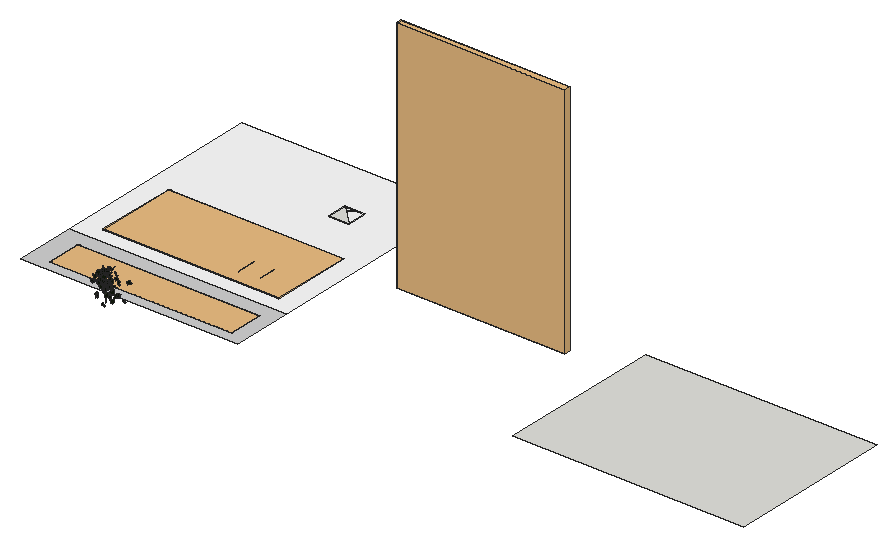
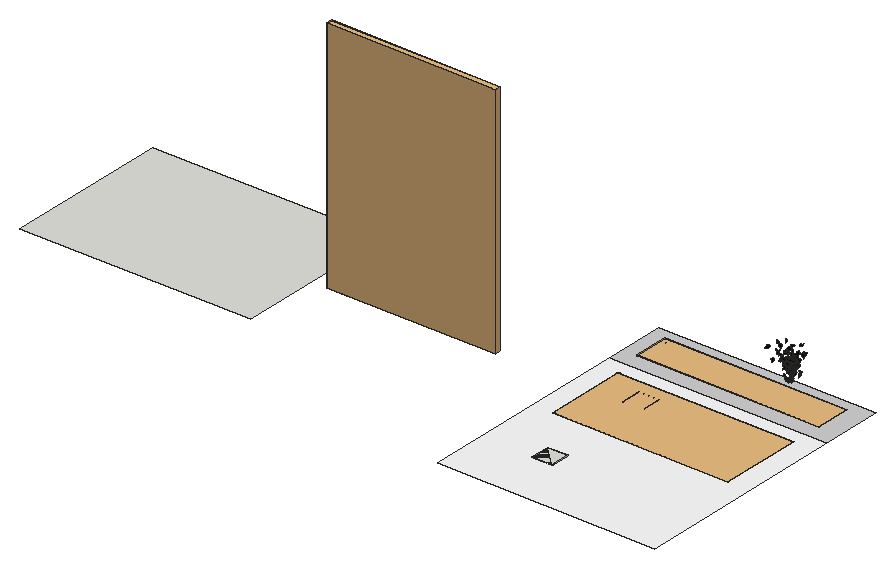
# SketchUp Ruby script. Lengths in inches.
U = 1.inch
M = Sketchup.active_model
def pt(a) = Geom::Point3d.new(a.map { |v| v * U })
def face(e, loops, mat)
  f = e.add_face(loops[0].map { |a| pt(a) })
  loops[1..].each { |l| e.add_face(l.map { |a| pt(a) }).erase! }
  f.material = f.back_material = mat if mat
  f
end
# faces: each face lists its corners as indices into pts; further lists are holes
def faces(e, pts, list, mat = nil) = list.each { |f| face(e, (f[0].is_a?(Array) ? f : [f]).map { |l| l.map { |i| pts[i] } }, mat) }
# xy, xz, yz: faces in a plane at the given z, y or x. An outline is a flat list of corners, or four numbers for a rectangle; further outlines are holes
def ring(l) = l.size == 4 ? [[l[0], l[1]], [l[2], l[1]], [l[2], l[3]], [l[0], l[3]]] : l.each_slice(2).to_a
def flat(e, list, mat, &to3) = list.each { |f| face(e, (f[0].is_a?(Array) ? f : [f]).map { |l| ring(l).map { |u, v| to3.(u, v) } }, mat) }
def xy(e, z, list, mat = nil) = flat(e, list, mat) { |x, y| [x, y, z] }
def xz(e, y, list, mat = nil) = flat(e, list, mat) { |x, z| [x, y, z] }
def yz(e, x, list, mat = nil) = flat(e, list, mat) { |y, z| [x, y, z] }
def lines(e, pts, list) = list.each { |a, b| e.add_line(pt(pts[a]), pt(pts[b])) }
# prism: a flat outline (further loops are holes) pulled along v
def prism(e, loops, v, mat = nil)
  f = face(e, loops, mat); d = Geom::Vector3d.new(v.map { |x| x * U })
  f.pushpull(f.normal.samedirection?(d) ? d.length : -d.length)
end
def box(e, o, s, mat = nil) = prism(e, [[o, [o[0] + s[0], o[1], o[2]], [o[0] + s[0], o[1] + s[1], o[2]], [o[0], o[1] + s[1], o[2]]]], [0, 0, s[2]], mat)
def at(x, y, z, deg = 0) = Geom::Transformation.translation(pt([x, y, z])) * Geom::Transformation.rotation(ORIGIN, Z_AXIS, deg.degrees)
def axes(o, x, y, z) = Geom::Transformation.new([*x, 0, *y, 0, *z, 0, *pt(o).to_a, 1])
def part(name) = M.definitions.add(name)
# library, detail: a bought-in or finely detailed component or shape, given as its bounding box
def library(name, o, s) = part(name).tap { |d| box(d.entities, o, s) }
def detail(e, o, s) = box(e.add_group.entities, o, s)
def put(e, d, t, mat = nil) = e.add_instance(d, t).tap { |i| i.material = mat if mat }
def group(e, t, mat = nil) = e.add_group.tap { |g| g.transformation = t; g.material = mat if mat }.entities
root = M.entities
M.materials.add("Concrete White 02 100cm").color = [209, 209, 209]
M.materials.add("Wall Paint White Semigloss 300cm").color = [255, 255, 255]
M.materials.add("efeu1").color = [18, 25, 13]
M.materials.add("efeu2").color = [43, 57, 29]
c1 = part("ivyleaf_10")
p = [[0,0.5,-0.03],[-0.0625,2.02,-0.43],[-0.19,2.01,-0.46],[-0.54,1.05,-0.29],[-0.52,0.625,-0.18],[-0.83,0.76,-0.28],
  [-1.16,0.64,-0.33],[-1.15,0.33,-0.24],[-0.77,-0.39,0.02],[-0.3,-0.51,0.16],[0.04,-0.48,0.23],[-0.02,2.01,-0.4375],
  [-0.06,2.01,-0.43],[0.04,-0.49,0.23],[0.67,-0.49,0.14],[1.38,0.36,-0.2],[1.375,0.51,-0.24],[0.81,0.65,-0.19],
  [0.62,0.59,-0.15],[0.6,1.09,-0.28],[0.5,1.23,-0.31]]
faces(c1.entities,p,[[0,1,2,3,4,5,6,7,8,9,10],[11,12,0,13,14,15,16,17,18,19,20]],"efeu2")
c2 = part("ivyleaf_9")
p = [[1.54,2.16,1.25],[1.36,2.04,1.19],[-0.21,0.99,0.68],[-0.71,1.11,0.82],[-0.85,0.86,0.67],[-0.8,0.17,0.21],
  [-0.9,-0.01,0.1],[-0.67,-0.16,-0.02],[-0.08,-0.08,-0.05],[-0.03,-0.6,-0.4],[0.65,-0.88,-0.66],[0.83,-0.6,-0.49],
  [1.29,-0.42,-0.43],[1.8125,-0.07,-0.26],[1.21,0.44,0.15]]
faces(c2.entities,p,[[0,1,2,3,4,5,6,7,8,9,10,11,12,13,14]],"efeu1")
c3 = library("Group\#7",[-0.5,-0.5,-0.1],[80.25,37.125,0.2])
c4 = library("Group\#21",[-0.5,-0.5,-0.1],[82.9375,15.8125,0.2])
c5 = part("Tlon Cubo 860 Ceiling 152 005")
xy(c5.entities,-3.04,[[-16.54,-16.54,-16.54,16.54,16.54,-16.54],[16.54,-16.54,-16.54,16.54,16.54,16.54]])
xy(c5.entities,0,[[-16.93,-16.93,16.93,-16.93,-16.93,16.93],[16.93,-16.93,16.93,16.93,-16.93,16.93]])
xz(c5.entities,-16.93,[[-16.93,-3.79,16.93,-3.79,-16.93,0],[16.93,-3.79,16.93,0,-16.93,0]])
xz(c5.entities,-16.3,[[-16.3,-3.66,-16.3,-3.24,16.3,-3.24],[-16.3,-3.66,16.3,-3.24,16.3,-3.66]])
xz(c5.entities,16.3,[[-16.3,-3.66,16.3,-3.24,-16.3,-3.24],[-16.3,-3.66,16.3,-3.66,16.3,-3.24]])
xz(c5.entities,16.93,[[-16.93,-3.79,-16.93,0,16.93,0],[-16.93,-3.79,16.93,0,16.93,-3.79]])
yz(c5.entities,-16.93,[[-16.93,-3.79,-16.93,0,16.93,0],[-16.93,-3.79,16.93,0,16.93,-3.79]])
yz(c5.entities,-16.3,[[-16.3,-3.66,16.3,-3.66,-16.3,-3.24],[16.3,-3.66,16.3,-3.24,-16.3,-3.24]])
yz(c5.entities,16.3,[[-16.3,-3.66,-16.3,-3.24,16.3,-3.66],[16.3,-3.66,-16.3,-3.24,16.3,-3.24]])
yz(c5.entities,16.93,[[-16.93,-3.79,16.93,-3.79,-16.93,0],[16.93,-3.79,16.93,0,-16.93,0]])
p = [[-16.93,-16.93,-3.79],[-16.93,16.93,-3.79],[-16.3,16.3,-3.66],[-16.3,-16.3,-3.66],[16.93,-16.93,-3.79],[16.3,-16.3,-3.66],
  [16.93,16.93,-3.79],[16.3,16.3,-3.66]]
faces(c5.entities,p,[[0,1,2],[2,3,0],[4,0,3],[3,5,4],[6,4,5],[5,7,6],[2,1,6],[6,7,2]])
c6 = library("Wall Panel 104-26",[-34.24,-2.8,0],[68.48,2.8,108.01])
xy(root,222.44,[[233.9,233.25,339.25,308.9375]])
xy(root,222.96,[[[17.04,223.4375,116.08,251.4375],[27.0625,229.01,109,243.82]],[29.0625,231.01,107,241.82]],"Concrete White 02 100cm")
xy(root,222.96,[[[17.04,251.4375,116.08,350],[27.28,259.07,106.53,295.19]],[29.26,261.05,104.55,293.21]],"Wall Paint White Semigloss 300cm")
put(root,c1,axes([54.74,225.27,223.34],[-0.39299,-0.30612,-0.04308],[0.03552,0.0245,-0.49813],[0.30708,-0.39458,0.00249]))
put(root,c2,axes([54.79,223.51,230.73],[0.15223,0.45595,-0.13759],[-0.04078,-0.13144,-0.48069],[-0.47451,0.15758,-0.00283]))
put(root,c1,axes([54.67,222.28,227.875],[0.18781,0.46033,-0.05313],[-0.06422,-0.03091,-0.49489],[-0.45891,0.19272,0.04751]))
put(root,c2,axes([54.63,224.2,230.9],[-0.23647,-0.43177,-0.08748],[0.0771,0.05719,-0.4907],[0.43375,-0.24556,0.03953]))
put(root,c2,axes([54.46,223.81,225.65],[-0.04401,0.01441,0.49785],[0.20399,-0.45543,0.03122],[0.45437,0.20586,0.03421]))
put(root,c1,axes([54.76,224.35,222.82],[-0.11813,0.47633,0.0957],[0.01873,-0.09395,0.49074],[0.48548,0.11952,0.00435]))
put(root,c1,axes([54.8125,223.74,229.92],[-0.16247,-0.45887,0.11419],[-0.03947,-0.10716,-0.48678],[0.47122,-0.16719,-0.0014]))
put(root,c2,axes([54.82,224.07,227.5],[0.33069,0.25026,-0.27931],[-0.27338,-0.09405,-0.40794],[-0.25672,0.42252,0.07463]))
put(root,c2,axes([54.93,222.97,231.93],[-0.41934,0.24934,-0.10946],[0.08858,-0.06515,-0.48776],[-0.2575,-0.42847,0.01047]))
put(root,c1,axes([54.4,224.44,229.78],[0.25917,0.01109,0.42744],[0.40933,0.13806,-0.25177],[-0.12361,0.48043,0.06248]))
put(root,c2,axes([54.91,223.96,227.22],[-0.01977,0.49756,0.04519],[0.00431,0.0454,-0.49792],[-0.49959,-0.0193,-0.00608]))
put(root,c2,axes([54.9,223.1,229.65],[-0.46927,-0.16626,-0.04625],[0.04,0.02555,-0.49774],[0.16787,-0.47085,-0.01068]))
put(root,c1,axes([54.53,225.04,225.03],[0.3416,-0.2445,0.27116],[0.29785,-0.02816,-0.40061],[0.21117,0.43523,0.12641]))
put(root,c1,axes([54.82,224.52,225.07],[-0.48477,0.12245,-0.00129],[0.00127,-0.00021,-0.5],[-0.12245,-0.48477,-0.00011]))
put(root,c1,axes([54.79,223.92,225.58],[0.13092,0.45702,0.15489],[-0.09873,0.18247,-0.45493],[-0.47235,0.08853,0.13802]))
put(root,c2,axes([54.43,220.97,227.32],[0.12677,-0.09783,0.47366],[0.46015,-0.12642,-0.14927],[0.14896,0.47376,0.05798]))
put(root,c2,axes([55.01,223.96,225.74],[-0.48818,-0.10682,-0.01641],[0.02228,-0.02522,-0.49887],[0.10575,-0.48781,0.02938]))
put(root,c1,axes([54.9,224.18,225.27],[0.05409,-0.49024,-0.08207],[0.00626,0.08322,-0.49299],[0.49703,0.0523,0.01514]))
put(root,c1,axes([54.68,223.84,227.29],[0.3283,-0.33192,-0.17903],[0.12633,-0.12686,0.46685],[-0.35533,-0.35177,0.00057]))
put(root,c2,axes([54.77,222.95,231.26],[0.42876,0.25458,-0.03677],[-0.0325,-0.01729,-0.49864],[-0.25517,0.42999,0.00173]))
put(root,c2,axes([54.68,221.82,229.07],[0.01874,-0.4987,0.03083],[0.06388,-0.0282,-0.4951],[0.49555,0.0225,0.06265]))
put(root,c2,axes([55.15,224.48,223.51],[-0.18777,0.42642,0.18141],[-0.0642,0.16991,-0.46584],[-0.45893,-0.19824,-0.00906]))
put(root,c2,axes([54.6,224,225.35],[0.34095,-0.36171,0.05399],[0.03558,-0.04066,-0.49707],[0.36399,0.3428,-0.00199]))
put(root,c2,axes([54.68,223.28,229.22],[-0.17881,-0.25855,-0.38882],[0.29211,0.26287,-0.30914],[0.36428,-0.33771,0.05704]))
put(root,c1,axes([55.07,223.97,223.26],[-0.00077,0.01495,0.49978],[-0.29049,0.40677,-0.01261],[-0.40696,-0.29037,0.00806]))
put(root,c1,axes([54.92,219.52,224.03],[0.07481,-0.47253,0.14532],[0.02935,-0.14247,-0.47837],[0.4935,0.0801,0.00642]))
put(root,c2,axes([54.71,222.47,225.48],[0.49795,0.03985,-0.02128],[-0.02127,-0.00101,-0.49955],[-0.03986,0.49841,0.00069]))
put(root,c2,axes([55.15,224.54,223.57],[-0.4649,0.17169,-0.06626],[0.05725,-0.03617,-0.49539],[-0.17491,-0.4682,0.01397]))
put(root,c1,axes([55,224.3125,225],[-0.42737,-0.25941,-0.00751],[0.00614,0.00437,-0.49994],[0.25945,-0.42742,-0.00055]))
put(root,c2,axes([55.25,223.5,230.83],[0.02618,0.18174,0.46507],[-0.34668,0.34177,-0.11404],[-0.35934,-0.31649,0.1439]))
put(root,c2,axes([54.84,223.68,229.86],[0.39661,0.2959,0.07172],[0.06573,0.03178,-0.49464],[-0.29728,0.40179,-0.0137]))
put(root,c1,axes([55.05,224.32,224.12],[-0.39858,-0.30158,-0.0136],[0.0106,0.00853,-0.49981],[0.3017,-0.39872,-0.00041]))
put(root,c2,axes([54.79,220.65,232.73],[0.33479,0.23997,0.28343],[0.2092,0.19343,-0.41088],[-0.30684,0.3937,0.02911]))
put(root,c2,axes([55.12,221.29,228.21],[0.17247,0.42585,-0.19724],[-0.11061,-0.16734,-0.458],[-0.45609,0.20162,0.03648]))
put(root,c1,axes([54.8,223.6,227.32],[-0.14284,-0.20554,0.43284],[0.22199,0.37188,0.24986],[-0.42464,0.26355,-0.01498]))
put(root,c1,axes([55.02,223.08,233.16],[-0.43688,0.24135,-0.02984],[0.02957,-0.00818,-0.49906],[-0.24138,-0.43782,-0.00712]))
put(root,c2,axes([54.82,223.34,230.75],[0.10441,-0.48052,-0.09058],[0.01782,0.09629,-0.49032],[0.48865,0.09916,0.03723]))
put(root,c2,axes([54.79,224.3,225.71],[0.38868,-0.31409,-0.01651],[-0.0047,0.02043,-0.49956],[0.31449,0.3885,0.01293]))
put(root,c2,axes([55.42,216.79,230.3125],[0.03331,-0.01586,0.49864],[-0.4223,0.26519,0.03664],[-0.26563,-0.42359,0.00427]))
put(root,c2,axes([55.05,224.22,224.61],[-0.11506,-0.461,0.1557],[-0.04092,-0.15026,-0.47513],[0.48486,-0.12208,-0.00315]))
put(root,c2,axes([54.93,224.35,230.43],[-0.03167,-0.01976,0.4986],[0.09113,-0.49144,-0.01369],[0.4906,0.09001,0.03473]))
put(root,c1,axes([55.24,221.85,226.79],[-0.2422,-0.41104,0.14961],[-0.04643,-0.1459,-0.47598],[0.43495,-0.24446,0.03251]))
put(root,c1,axes([55.24,221.74,227.29],[-0.14093,-0.47072,0.09253],[-0.0412,-0.08421,-0.49113],[0.47796,-0.14606,-0.01505]))
put(root,c2,axes([54.93,220.98,230.6],[0.28595,0.1642,0.37586],[0.27675,0.26092,-0.32454],[-0.30272,0.39364,0.05834]))
put(root,c2,axes([55.08,220.375,232.59],[-0.26685,-0.32602,-0.26926],[0.16804,0.21041,-0.4213],[0.38801,-0.31534,-0.00273]))
put(root,c2,axes([54.92,220.29,223.23],[0.01995,-0.0013,-0.4996],[0.48199,-0.13153,0.01959],[-0.13147,-0.48239,-0.00399]))
put(root,c2,axes([55.07,224.36,223.47],[0.05722,-0.48644,0.10052],[0.00946,-0.1001,-0.48979],[0.49663,0.05795,-0.00225]))
put(root,c2,axes([55.11,224.3,225.38],[-0.17615,-0.39077,-0.25743],[0.19775,0.18713,-0.41938],[0.42411,-0.24955,0.08862]))
put(root,c2,axes([54.86,219.76,228.9375],[0.24319,-0.12501,0.41861],[0.39107,-0.15126,-0.27237],[0.19473,0.45988,0.02421]))
put(root,c2,axes([54.97,222.42,225.1],[0.13551,-0.00464,0.48127],[0.46789,0.11843,-0.1306],[-0.11278,0.48575,0.03644]))
put(root,c2,axes([55.44,216.93,230.34],[0.24636,0.28864,-0.32557],[-0.21268,-0.2465,-0.37948],[-0.37957,0.32546,0.00132]))
put(root,c2,axes([55.22,224.14,227.51],[-0.1188,0.06348,-0.48152],[0.38822,-0.28546,-0.13341],[-0.29184,-0.40557,0.01854]))
put(root,c2,axes([55.05,224.45,223.52],[0.34332,0.12961,0.33961],[0.29917,0.16458,-0.36525],[-0.20647,0.454,0.03546]))
put(root,c2,axes([55.02,223.84,226.94],[-0.00669,-0.01745,0.49965],[0.49902,-0.03082,0.00561],[0.0306,0.49874,0.01783]))
put(root,c2,axes([55.01,221.59,230.28],[0.07076,0.0815,-0.48821],[0.30969,0.37743,0.10789],[0.38612,-0.31765,0.00294]))
put(root,c2,axes([55.07,222.66,229.26],[-0.07433,-0.04638,-0.49226],[0.48626,0.08332,-0.08128],[0.08957,-0.49082,0.03272]))
put(root,c2,axes([55.05,222.25,224.99],[0.28566,-0.35628,0.20363],[0.14536,-0.14417,-0.45616],[0.38376,0.31981,0.02121]))
put(root,c2,axes([55.1,224.54,223.55],[0.46834,0.03239,0.17206],[0.16767,0.05851,-0.4674],[-0.05041,0.49551,0.04395]))
put(root,c2,axes([55.23,224.46,231.42],[-0.16371,-0.21828,-0.41899],[0.24238,0.34182,-0.27278],[0.40552,-0.29243,-0.0061]))
put(root,c2,axes([55.2,221.875,227],[0.04063,-0.39508,-0.30374],[0.1157,0.3039,-0.37981],[0.48473,-0.03942,0.11611]))
put(root,c2,axes([55.75,225.38,222.97],[-0.05641,0.18267,0.46201],[-0.15665,0.43472,-0.19101],[-0.47147,-0.16629,0.00819]))
put(root,c2,axes([55.86,224.24,230.53],[-0.41447,0.14918,-0.23655],[0.21847,-0.09132,-0.44038],[-0.1746,-0.46841,0.01052]))
put(root,c1,axes([55.62,223.13,222.875],[0.19913,0.23265,-0.39525],[0.21258,0.33499,0.30429],[0.4064,-0.28922,0.0345]))
put(root,c1,axes([55.84,224.88,226.45],[0.38342,0.23659,-0.21682],[-0.18295,-0.1164,-0.45053],[-0.26366,0.42483,-0.0027]))
put(root,c2,axes([56,218.0625,223.36],[0.00937,0.31919,0.38475],[0.00962,0.38463,-0.31933],[-0.49982,0.01338,0.00107]))
put(root,c1,axes([56.375,225.89,223.95],[-0.20535,0.03273,0.45471],[-0.4497,0.06734,-0.20793],[-0.07485,-0.49436,0.00178]))
put(root,c2,axes([56.16,224.24,231.68],[-0.17568,0.46515,-0.05263],[-0.01931,0.04897,0.49722],[0.46772,0.17673,0.00076]))
put(root,c2,axes([56.27,220.23,230.11],[0.16897,-0.18249,-0.43376],[-0.26334,0.34528,-0.24786],[0.39,0.31221,0.02057]))
put(root,c2,axes([56.14,224.73,229.74],[0.13843,0.11469,0.46657],[0.35026,0.30826,-0.1797],[-0.32887,0.37659,0.005]))
put(root,c2,axes([56.52,224.8,232.04],[-0.08588,0.48461,-0.08817],[0.0105,-0.08768,-0.49214],[-0.49246,-0.08638,0.00488]))
put(root,c2,axes([56.65,223.52,224.83],[0.09256,-0.18019,0.45713],[-0.13385,0.43833,0.19988],[-0.47278,-0.15937,0.0329]))
put(root,c2,axes([56.28,224.26,229.26],[0.43042,0.18176,0.17804],[0.1591,0.08077,-0.46708],[-0.19856,0.45874,0.0117]))
put(root,c2,axes([56.24,221.89,224.15],[0.10665,-0.12534,0.47214],[0.41759,-0.22736,-0.15468],[0.25347,0.42731,0.05619]))
put(root,c1,axes([56.64,224.33,230.26],[-0.14665,0.17664,0.44417],[0.26871,-0.35378,0.22942],[0.39533,0.306,0.00884]))
put(root,c1,axes([56.71,224.18,232.61],[-0.2931,0.26784,0.3039],[0.21623,-0.21375,0.39693],[0.34255,0.3641,0.00947]))
put(root,c2,axes([56.58,224.26,227.34],[-0.17966,-0.14719,-0.44278],[0.34241,0.28073,-0.23226],[0.31698,-0.38668,-0.00008]))
put(root,c2,axes([57.22,216.16,233.12],[-0.2476,-0.41616,-0.1245],[-0.04546,-0.11769,0.48382],[-0.432,0.25091,0.02044]))
put(root,c2,axes([56.85,221.54,233.34],[-0.07757,-0.03678,-0.49258],[0.4933,-0.03128,-0.07535],[-0.02527,-0.49766,0.04114]))
put(root,c1,axes([56.84,224.32,228.99],[0.08704,0.01306,-0.49219],[0.47168,0.14114,0.08716],[0.14122,-0.47949,0.01225]))
put(root,c2,axes([57.19,221.27,225.92],[-0.06228,-0.0934,0.48723],[0.31107,0.37519,0.11168],[-0.38647,0.31704,0.01138]))
put(root,c2,axes([57.2,223.66,226.4],[0.44863,-0.15315,0.15898],[-0.14396,0.07001,0.47368],[-0.16735,-0.47079,0.01872]))
put(root,c2,axes([57.29,225.67,231.82],[-0.14493,0.34031,-0.33643],[-0.12988,0.31035,0.36988],[0.46057,0.1946,-0.00156]))
put(root,c2,axes([57.4,219.7,229.85],[-0.23092,0.06367,-0.43889],[0.42451,-0.11146,-0.23953],[-0.12834,-0.48324,-0.00258]))
put(root,c2,axes([57.63,217.6875,230.08],[-0.07111,-0.23967,0.43301],[-0.0715,-0.4279,-0.24858],[0.48972,-0.09728,0.02658]))
put(root,c2,axes([57.77,219.93,229.07],[0.13188,0.33575,0.34623],[0.10213,0.33136,-0.36024],[-0.47135,0.16574,0.01882]))
put(root,c2,axes([57.77,218.72,228.21],[-0.11729,-0.4334,0.22003],[-0.04165,-0.21655,-0.44875],[0.48426,-0.12359,0.0147]))
put(root,c2,axes([57.85,220.89,231.52],[-0.20636,0.14672,-0.43115],[0.34974,-0.25213,-0.2532],[-0.29171,-0.40608,0.00143]))
put(root,c2,axes([57.88,223.75,227.08],[-0.15766,0.04954,-0.4719],[0.45483,-0.12591,-0.16517],[-0.1352,-0.48134,-0.00537]))
put(root,c2,axes([58.38,222.88,229.6],[-0.04313,-0.0259,0.49746],[0.30656,0.39219,0.047],[-0.39263,0.30906,-0.01795]))
put(root,c2,axes([58.625,220.9375,233.54],[0.15103,0.47626,0.01923],[0.00562,0.0184,-0.49963],[-0.47661,0.15113,0.00021]))
put(root,c2,axes([58.93,219.91,226.7],[-0.41609,0.15166,-0.2321],[-0.22217,0.06803,0.44273],[0.16587,0.47156,0.01078]))
put(root,c2,axes([58.43,222.28,232.03],[-0.07367,-0.02368,-0.49398],[0.49383,0.02334,-0.07477],[0.0266,-0.49889,0.01995]))
put(root,c2,axes([59.125,223.34,223.56],[-0.32921,0.1168,-0.35774],[0.33635,-0.12185,-0.34932],[-0.16878,-0.47065,0.00166]))
put(root,c2,axes([59.07,219.63,227.22],[0.14632,-0.09642,-0.46829],[0.37289,-0.28349,0.17489],[-0.29924,-0.40042,-0.01105]))
put(root,c2,axes([59.28,224.98,231.29],[0.40123,-0.20133,-0.22019],[-0.19847,0.09541,-0.44889],[0.22277,0.44762,-0.00335]))
put(root,c2,axes([59.58,218.14,233.18],[-0.22374,-0.37601,-0.24198],[0.1356,0.20079,-0.43737],[0.42609,-0.26135,0.01212]))
put(root,c2,axes([59.6,219.05,223.36],[-0.17017,0.04136,-0.46833],[0.45333,-0.11759,-0.1751],[-0.12463,-0.48421,0.00252]))
put(root,c2,axes([60.2,218.55,224.85],[-0.2996,-0.14525,0.37302],[0.33069,0.17275,0.33286],[-0.22557,0.44616,-0.00745]))
put(root,c2,axes([60.27,221.35,225.31],[0.24495,0.33587,0.27783],[0.15116,0.23347,-0.4155],[-0.40884,0.28755,0.01283]))
put(root,c2,axes([60.37,220.3,223.55],[-0.1779,0.29268,0.36427],[0.18367,-0.3146,0.34248],[0.42967,0.25566,0.00442]))
put(root,c2,axes([60.62,220.56,231.58],[-0.12098,-0.23483,0.42452],[-0.08962,-0.41917,-0.25742],[0.47679,-0.13837,0.05933]))
put(root,c2,axes([60.71,220.54,230.8125],[-0.01221,-0.30517,-0.39588],[0.15534,0.37407,-0.29315],[0.4751,-0.13015,0.08568]))
put(root,c2,axes([60.87,215.8125,222.78],[0.4597,-0.15751,0.11773],[-0.10257,0.06336,0.48525],[-0.16779,-0.47029,0.02594]))
put(root,c2,axes([61.18,220.95,226.39],[0.02875,-0.17837,0.46622],[-0.08126,0.45909,0.18065],[-0.49251,-0.08616,-0.00259]))
put(root,c2,axes([61.11,221.23,228.26],[0.48388,0.11419,0.0531],[0.0516,0.01257,-0.49717],[-0.11488,0.48662,0.00038]))
put(root,c2,axes([61.47,220.13,225.98],[-0.26953,-0.02657,0.4203],[0.41901,-0.06696,0.26447],[0.04223,0.49478,0.05836]))
put(root,c2,axes([62.09,218.02,229.55],[0.27563,0.1863,-0.37325],[0.31125,0.20603,0.33268],[0.27776,-0.41574,-0.00239]))
put(root,c2,axes([63.54,220.0625,232.78],[0.25221,0.21283,-0.37562],[-0.32542,-0.19215,-0.32738],[-0.2837,0.40961,0.0416]))
put(root,c2,axes([63.86,217.82,224.38],[-0.31765,-0.37023,-0.10969],[-0.07157,-0.08313,0.48782],[-0.37945,0.32561,-0.00019]))
put(root,c2,axes([63.84,216.42,232.3],[-0.01885,-0.16576,0.47135],[0.11075,-0.46134,-0.15781],[0.48722,0.09845,0.05411]))
put(root,c2,axes([65.49,218.0625,227.23],[-0.44331,-0.21402,0.08761],[-0.07313,-0.04996,-0.49209],[0.21939,-0.44911,0.01299]))
put(root,c2,axes([65.63,218.63,232.76],[-0.18475,-0.03412,-0.46336],[0.45218,0.10139,-0.18776],[0.10677,-0.48842,-0.00661]))
put(root,c2,axes([66.47,217.84,227.63],[-0.12246,-0.14289,0.46324],[-0.15386,-0.44163,-0.17689],[0.45971,-0.18587,0.06419]))
put(root,c2,axes([66.67,217.79,227.61],[-0.10675,0.11156,0.47556],[0.24775,-0.40716,0.15113],[0.42098,0.2679,0.03165]))
put(root,c3,at(27.28,259.07,222.96))
put(root,c2,axes([67.15,219.85,224.88],[0.16968,-0.22974,0.4104],[0.27789,-0.30302,-0.28453],[0.37946,0.32465,0.02485]))
put(root,c2,axes([67.53,221.89,231.8],[0.00266,-0.00923,-0.49991],[0.13566,0.48118,-0.00816],[0.48124,-0.13559,0.00506]))
put(root,c4,at(27.0625,229.01,222.96))
put(root,c5,axes([87.9,269.25,222.96],[0.2697,0,0],[0,0.2697,0],[0,0,0.2697]))
put(root,c5,axes([87.9,320.87,222.96],[0.2697,0,0],[0,0.2697,0],[0,0,0.2697]))
put(root,c6,axes([180.6875,284.3125,229.74],[1.1252,0,0],[0,1,0],[0,0,1]))
